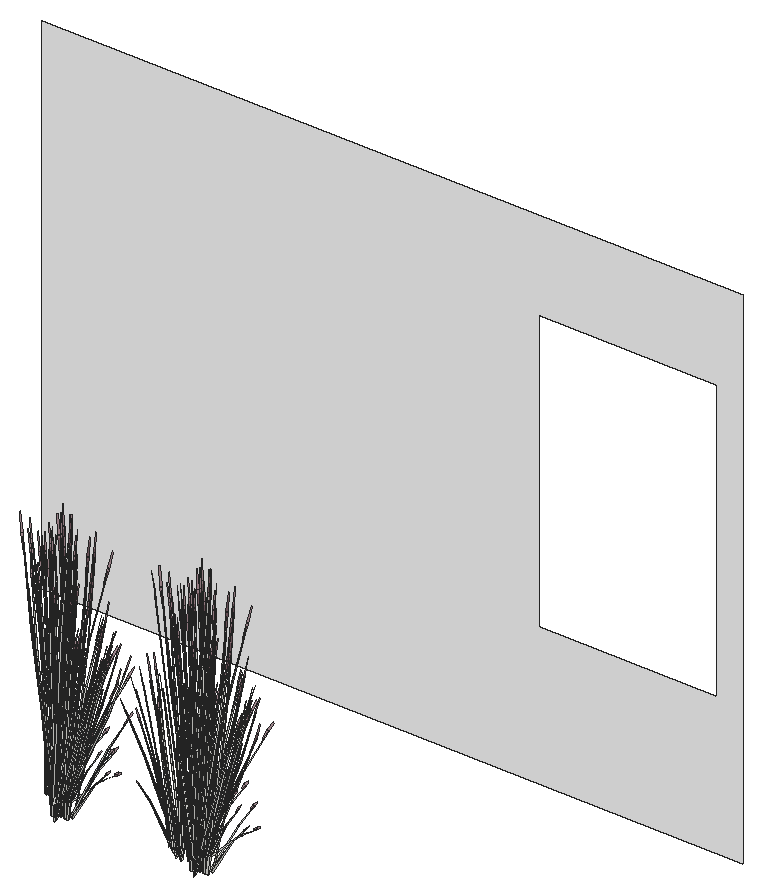
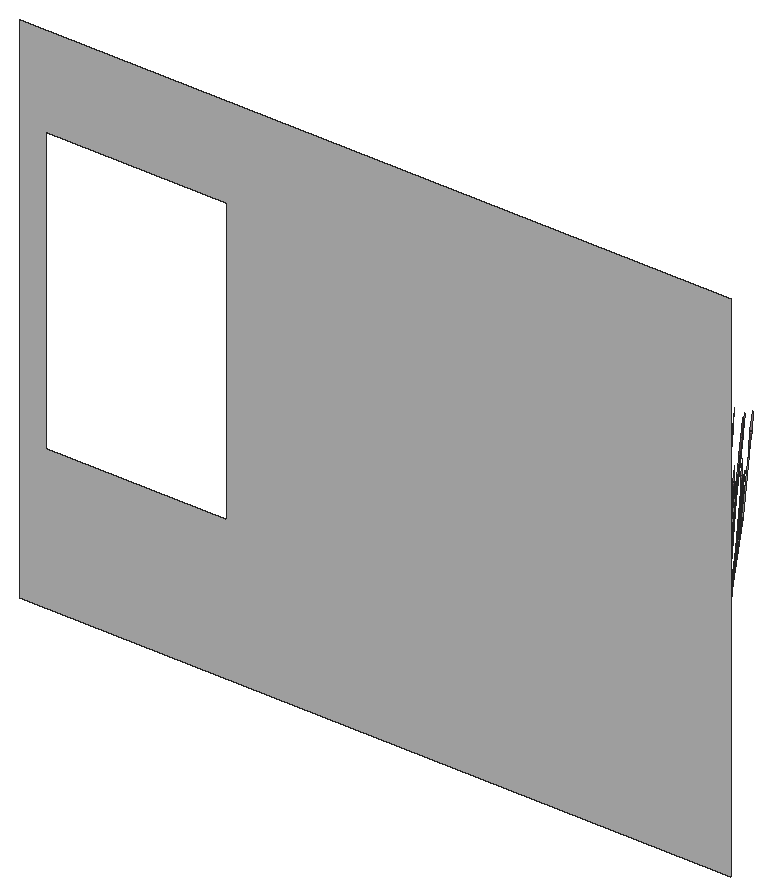
# SketchUp Ruby script. Lengths in inches.
U = 1.inch
M = Sketchup.active_model
def pt(a) = Geom::Point3d.new(a.map { |v| v * U })
def face(e, loops, mat)
  f = e.add_face(loops[0].map { |a| pt(a) })
  loops[1..].each { |l| e.add_face(l.map { |a| pt(a) }).erase! }
  f.material = f.back_material = mat if mat
  f
end
# faces: each face lists its corners as indices into pts; further lists are holes
def faces(e, pts, list, mat = nil) = list.each { |f| face(e, (f[0].is_a?(Array) ? f : [f]).map { |l| l.map { |i| pts[i] } }, mat) }
# xy, xz, yz: faces in a plane at the given z, y or x. An outline is a flat list of corners, or four numbers for a rectangle; further outlines are holes
def ring(l) = l.size == 4 ? [[l[0], l[1]], [l[2], l[1]], [l[2], l[3]], [l[0], l[3]]] : l.each_slice(2).to_a
def flat(e, list, mat, &to3) = list.each { |f| face(e, (f[0].is_a?(Array) ? f : [f]).map { |l| ring(l).map { |u, v| to3.(u, v) } }, mat) }
def xy(e, z, list, mat = nil) = flat(e, list, mat) { |x, y| [x, y, z] }
def xz(e, y, list, mat = nil) = flat(e, list, mat) { |x, z| [x, y, z] }
def yz(e, x, list, mat = nil) = flat(e, list, mat) { |y, z| [x, y, z] }
def lines(e, pts, list) = list.each { |a, b| e.add_line(pt(pts[a]), pt(pts[b])) }
# prism: a flat outline (further loops are holes) pulled along v
def prism(e, loops, v, mat = nil)
  f = face(e, loops, mat); d = Geom::Vector3d.new(v.map { |x| x * U })
  f.pushpull(f.normal.samedirection?(d) ? d.length : -d.length)
end
def box(e, o, s, mat = nil) = prism(e, [[o, [o[0] + s[0], o[1], o[2]], [o[0] + s[0], o[1] + s[1], o[2]], [o[0], o[1] + s[1], o[2]]]], [0, 0, s[2]], mat)
def at(x, y, z, deg = 0) = Geom::Transformation.translation(pt([x, y, z])) * Geom::Transformation.rotation(ORIGIN, Z_AXIS, deg.degrees)
def axes(o, x, y, z) = Geom::Transformation.new([*x, 0, *y, 0, *z, 0, *pt(o).to_a, 1])
def part(name) = M.definitions.add(name)
# library, detail: a bought-in or finely detailed component or shape, given as its bounding box
def library(name, o, s) = part(name).tap { |d| box(d.entities, o, s) }
def detail(e, o, s) = box(e.add_group.entities, o, s)
def put(e, d, t, mat = nil) = e.add_instance(d, t).tap { |i| i.material = mat if mat }
def group(e, t, mat = nil) = e.add_group.tap { |g| g.transformation = t; g.material = mat if mat }.entities
root = M.entities
M.materials.add("LightPink_Translucent").color = [144, 107, 117]
M.materials["LightPink_Translucent"].alpha = 0.75
M.materials.add("M00_Soft_Cloud").color = [255, 255, 255]
c1 = part("blade")
p = [[2.15,0.21,22],[0,0.17,0],[0.09,0.45,0],[2.18,0.31,22],[2.29,0.31,22],[0.38,0.45,0],
  [2.48,0.24,33],[2.49,0.24,33],[2.48,0.22,33]]
faces(c1.entities,p,[[0,1,2,3],[4,5,2,3],[6,3,4,7],[8,0,3,6]])
c2 = part("seeds")
p = [[0.3,-0.1,1.38],[-0.01,-0.03,1.59],[-0.01,-0.03,0.03],[0.14,-0.07,-0.07],[0.29,-0.03,3],[0.15,0.01,3.11]]
faces(c2.entities,p,[[0,1,2,3],[1,0,4,5]],"LightPink_Translucent")
c3 = part("blade with seeds")
put(c3.entities,c1,at(0,0,0))
put(c3.entities,c2,axes([2.4,0.25,30.99],[1.5799,-0.05474,1.17369],[-0.12525,1.92788,0.29478],[-0.07173,-0.02425,1.56792]))
xz(root,72.98,[[[234,0,399,120],[351,33,393,99]]],"M00_Soft_Cloud")
put(root,c3,axes([286.19,11.56,-3.97],[0.17848,0.53243,-0.30978],[-0.70886,0.15119,0.30978],[0.1429,0.0614,1.38974]))
put(root,c3,axes([318.98,11.56,-3.97],[0.17848,0.53243,-0.30978],[-0.70886,0.15119,0.30978],[0.1429,0.0614,1.38974]))
put(root,c3,axes([287.41,13.6875,-1.27],[0.27906,0.41663,0.0643],[-0.50888,0.20393,0.50621],[0.22432,-0.04024,0.77189]))
put(root,c3,axes([320.2,13.6875,-1.27],[0.27906,0.41663,0.0643],[-0.50888,0.20393,0.50621],[0.22432,-0.04024,0.77189]))
put(root,c3,axes([284.76,12.75,-3.62],[-0.96033,-0.12874,0.49198],[0.19544,-0.7271,0.19306],[0.14034,0.07021,1.70813]))
put(root,c3,axes([317.56,12.75,-3.62],[-0.96033,-0.12874,0.49198],[0.19544,-0.7271,0.19306],[0.14034,0.07021,1.70813]))
put(root,c3,axes([287.36,13.54,-1.27],[-0.21466,0.55714,0.48003],[-0.70573,-0.19051,0.3958],[0.27753,-0.03348,0.9933]))
put(root,c3,axes([320.15,13.54,-1.27],[-0.21466,0.55714,0.48003],[-0.70573,-0.19051,0.3958],[0.27753,-0.03348,0.9933]))
put(root,c3,axes([284,14.55,-3.8],[-0.24791,-0.5268,0],[0.70791,-0.18448,0],[0,0,1.54371]))
put(root,c3,axes([316.79,14.55,-3.8],[-0.24791,-0.5268,0],[0.70791,-0.18448,0],[0,0,1.54371]))
put(root,c3,axes([283.52,14.05,-3.38],[-0.14658,0.54532,0.1448],[-0.71613,-0.09466,-0.41347],[-0.13033,-0.05599,1.26744]))
put(root,c3,axes([316.32,14.05,-3.38],[-0.14658,0.54532,0.1448],[-0.71613,-0.09466,-0.41347],[-0.13033,-0.05599,1.26744]))
put(root,c3,axes([313.54,12.63,-0.95],[0.63144,0.17046,0.35414],[-0.18417,0.49731,-0.4572],[-0.25423,0.0456,0.87481]))
put(root,c3,axes([284.93,14.47,-3.82],[0.79769,-0.20732,-0.19198],[0.2803,0.59721,0.00008],[0.08805,-0.02292,1.73897]))
put(root,c3,axes([317.72,14.47,-3.82],[0.79769,-0.20732,-0.19198],[0.2803,0.59721,0.00008],[0.08805,-0.02292,1.73897]))
put(root,c3,axes([285.2,14.72,-3.53],[0.21949,-0.60727,0.17642],[0.8032,0.17185,0.35086],[-0.13875,0.00296,1.60407]))
put(root,c3,axes([318,14.72,-3.53],[0.21949,-0.60727,0.17642],[0.8032,0.17185,0.35086],[-0.13875,0.00296,1.60407]))
put(root,c3,axes([285.02,13.34,-3.79],[0.53038,0.39469,0],[-0.53038,0.39469,0],[0,0,1.69266]))
put(root,c3,axes([317.8125,13.34,-3.79],[0.53038,0.39469,0],[-0.53038,0.39469,0],[0,0,1.69266]))
put(root,c3,axes([314.8,12.6,-2.66],[0.21597,-0.08839,1.77064],[0.07448,0.61717,0.13857],[-0.4678,0.08189,0.63284]))
put(root,c3,axes([286.46,13.17,-3.53],[-0.59697,-0.44509,0.17642],[0.60159,-0.4317,0.35086],[-0.06593,0.0909,1.60407]))
put(root,c3,axes([319.25,13.17,-3.53],[-0.59697,-0.44509,0.17642],[0.60159,-0.4317,0.35086],[-0.06593,0.0909,1.60407]))
put(root,c3,axes([285.35,12.5,-3.94],[0.79037,0.10018,-0.62353],[-0.16679,0.61794,-0.16365],[0.23587,0.07488,1.37633]))
put(root,c3,axes([318.14,12.5,-3.94],[0.79037,0.10018,-0.62353],[-0.16679,0.61794,-0.16365],[0.23587,0.07488,1.37633]))
put(root,c3,axes([288.84,13.58,-3.23],[-0.46945,0.10088,1.1486],[0.22097,-0.4169,0.84392],[0.24904,0.02853,0.25299]))
put(root,c3,axes([321.64,13.58,-3.23],[-0.46945,0.10088,1.1486],[0.22097,-0.4169,0.84392],[0.24904,0.02853,0.25299]))
put(root,c3,axes([283.82,14.78,-3.8],[-0.76598,-0.27433,0],[0.36864,-0.57001,0],[0,0,1.62707]))
put(root,c3,axes([316.62,14.78,-3.8],[-0.76598,-0.27433,0],[0.36864,-0.57001,0],[0,0,1.62707]))
put(root,c3,axes([284.46,14.05,-3.54],[-0.74193,-0.49181,-0.25192],[0.6243,-0.55226,0.5513],[-0.19979,0.05753,1.68216]))
put(root,c3,axes([317.25,14.05,-3.54],[-0.74193,-0.49181,-0.25192],[0.6243,-0.55226,0.5513],[-0.19979,0.05753,1.68216]))
put(root,c3,axes([282.51,15,-3.52],[0.7111,0.30552,0.49651],[-0.42504,0.54784,0],[-0.16196,-0.06958,1.57504]))
put(root,c3,axes([315.3,15,-3.52],[0.7111,0.30552,0.49651],[-0.42504,0.54784,0],[-0.16196,-0.06958,1.57504]))
put(root,c3,axes([285.01,12.88,-3.28],[0.36864,-0.55059,0.44739],[0.76598,0.26498,-0.21531],[0,0.12692,1.43643]))
put(root,c3,axes([317.81,12.88,-3.28],[0.36864,-0.55059,0.44739],[0.76598,0.26498,-0.21531],[0,0.12692,1.43643]))
put(root,c3,axes([288.625,15.34,-1.29],[-0.0687,-0.05349,1.77383],[0.15029,-0.57341,-0.16761],[0.27062,-0.03664,0.31391]))
put(root,c3,axes([312.48,13.02,-1.28],[-0.12407,0.07933,1.74944],[0.01055,0.57963,-0.27667],[-0.2844,0.07538,0.14031]))
put(root,c3,axes([284.87,13.2,-3.71],[0,0.70667,-0.05637],[-0.95008,0,0],[0,0.02221,1.79368]))
put(root,c3,axes([317.66,13.2,-3.71],[0,0.70667,-0.05637],[-0.95008,0,0],[0,0.02221,1.79368]))
put(root,c3,axes([313.31,12.94,-1.32],[-0.20584,0.55581,-0.51099],[-0.70573,-0.19051,-0.3958],[-0.28414,0.05097,0.97773]))
put(root,c3,axes([313.27,12.46,-0.97],[0.38229,0.5533,-0.1216],[-0.6785,0.2719,-0.67495],[-0.28593,0.073,1.02557]))
put(root,c3,axes([284.94,12.7,-3.79],[0.45644,0.51287,-0.44739],[-0.69137,0.36116,0.21531],[0.14771,0.06346,1.43643]))
put(root,c3,axes([317.73,12.7,-3.79],[0.45644,0.51287,-0.44739],[-0.69137,0.36116,0.21531],[0.14771,0.06346,1.43643]))
put(root,c3,axes([288.03,14.87,-2.07],[-0.14542,-0.51365,-0.03492],[0.68734,-0.11809,-0.15832],[0.14353,0.03256,0.52218]))
put(root,c3,axes([320.82,14.87,-2.07],[-0.14542,-0.51365,-0.03492],[0.68734,-0.11809,-0.15832],[0.14353,0.03256,0.52218]))
put(root,c3,axes([314.89,15.32,-3.625],[-0.47504,0.61229,0],[-0.79476,-0.34146,-0.51607],[-0.18101,-0.07777,1.63711]))
put(root,c3,axes([286.25,14.85,-0.97],[0.04068,-0.62141,-0.1216],[0.77029,0.01698,-0.67495],[0.29667,0.04317,1.02557]))
put(root,c3,axes([319.04,14.85,-0.97],[0.04068,-0.62141,-0.1216],[0.77029,0.01698,-0.67495],[0.29667,0.04317,1.02557]))
put(root,c3,axes([286.95,13.19,-3.52],[0,-0.61104,0.49651],[0.85008,0,0],[0,0.13917,1.57504]))
put(root,c3,axes([319.74,13.19,-3.52],[0,-0.61104,0.49651],[0.85008,0,0],[0,0.13917,1.57504]))
put(root,c3,axes([284.82,13.65,-3.28],[0.82508,-0.03772,0.44739],[0.07462,0.62614,-0.21531],[-0.14771,0.06346,1.43643]))
put(root,c3,axes([317.61,13.65,-3.28],[0.82508,-0.03772,0.44739],[0.07462,0.62614,-0.21531],[-0.14771,0.06346,1.43643]))
put(root,c3,axes([285.33,13.01,-3.38],[0.70791,-0.1782,0.1448],[0.24791,0.50885,-0.41347],[0,0.11199,1.26744]))
put(root,c3,axes([318.125,13.01,-3.38],[0.70791,-0.1782,0.1448],[0.24791,0.50885,-0.41347],[0,0.11199,1.26744]))
put(root,c3,axes([286.13,14.61,-0.95],[-0.43232,-0.38257,0.35414],[0.49364,-0.36215,-0.4572],[0.25081,0.0551,0.87481]))
put(root,c3,axes([318.92,14.61,-0.95],[-0.43232,-0.38257,0.35414],[0.49364,-0.36215,-0.4572],[0.25081,0.0551,0.87481]))
put(root,c3,axes([284.08,13.95,-3.79],[-0.82508,0.03772,-0.44739],[-0.07462,-0.62614,0.21531],[-0.14771,0.06346,1.43643]))
put(root,c3,axes([316.875,13.95,-3.79],[-0.82508,0.03772,-0.44739],[-0.07462,-0.62614,0.21531],[-0.14771,0.06346,1.43643]))
put(root,c3,axes([287.96,14.25,-3.41],[-0.18299,-0.15028,1.43002],[0.23809,-0.49714,-0.30754],[0.37023,0.06735,0.61141]))
put(root,c3,axes([284.69,14.8,-3.8],[0.76598,0.27433,0],[-0.36864,0.57001,0],[0,0,1.74954]))
put(root,c3,axes([317.49,14.8,-3.8],[0.76598,0.27433,0],[-0.36864,0.57001,0],[0,0,1.74954]))
put(root,c3,axes([286.92,14.48,-1.28],[0.16299,-0.01033,1.74944],[0.44707,-0.47471,-0.27667],[0.28992,0.06266,0.14031]))
put(root,c3,axes([319.71,14.48,-1.28],[0.16299,-0.01033,1.74944],[0.44707,-0.47471,-0.27667],[0.28992,0.06266,0.14031]))
put(root,c3,axes([285,15.4,-3.81],[-0.46912,-0.61443,-0.05142],[0.79476,-0.34146,0.51607],[-0.19584,0.0585,1.6363]))
put(root,c3,axes([317.79,15.4,-3.81],[-0.46912,-0.61443,-0.05142],[0.79476,-0.34146,0.51607],[-0.19584,0.0585,1.6363]))
put(root,c3,axes([284.83,13.92,-3.38],[0.56134,0.36712,0.1448],[-0.46823,0.41419,-0.41347],[-0.13033,0.05599,1.26744]))
put(root,c3,axes([317.625,13.92,-3.38],[0.56134,0.36712,0.1448],[-0.46823,0.41419,-0.41347],[-0.13033,0.05599,1.26744]))
put(root,c3,axes([313.19,14.01,-1.27],[-0.18844,-0.56237,0.48003],[0.73919,-0.0976,0.3958],[-0.21785,0.13226,0.9933]))
put(root,c3,axes([313.05,13.9,-1.27],[-0.52161,-0.25698,0.0643],[0.30368,-0.36595,0.50621],[-0.16723,0.11831,0.77189]))
put(root,c3,axes([313.28,13.23,-2.125],[0.26363,-0.12925,1.71376],[0.22195,0.59723,0.13857],[-0.41388,0.13498,0.73262]))
put(root,c3,axes([286.28,14.55,-1.02],[0.75952,0.01471,-0.71045],[-0.05101,0.61953,0.08574],[0.32177,0.06538,1.00501]))
put(root,c3,axes([285.43,15.05,-3.52],[0.7111,-0.30552,0.49651],[0.42504,0.54784,0],[-0.16196,0.06958,1.57504]))
put(root,c3,axes([318.22,15.05,-3.52],[0.7111,-0.30552,0.49651],[0.42504,0.54784,0],[-0.16196,0.06958,1.57504]))
put(root,c3,axes([284.42,14.57,-3.71],[0.33034,0.70197,-0.06012],[-0.94388,0.24598,0],[0.01154,0.02451,1.72173]))
put(root,c3,axes([317.21,14.57,-3.71],[0.33034,0.70197,-0.06012],[-0.94388,0.24598,0],[0.01154,0.02451,1.72173]))
put(root,c3,axes([284.78,15.32,-3.97],[-0.70886,-0.15119,-0.30978],[0.17848,-0.53243,0.30978],[-0.1429,0.0614,1.38974]))
put(root,c3,axes([317.58,15.32,-3.97],[-0.70886,-0.15119,-0.30978],[0.17848,-0.53243,0.30978],[-0.1429,0.0614,1.38974]))
put(root,c3,axes([312.46,14.24,-3.41],[0.26405,0.05016,1.43002],[0.17019,0.51235,-0.30754],[-0.35868,0.0959,0.61141]))
put(root,c3,axes([313.65,13.83,-0.95],[0.66138,-0.08733,0.35414],[0.17464,0.49921,-0.4572],[-0.18953,0.13408,0.87481]))
put(root,c3,axes([287.52,13.29,-3.625],[0.95008,0,0],[0,0.68292,-0.51607],[0,0.15554,1.63711]))
put(root,c3,axes([320.32,13.29,-3.625],[0.95008,0,0],[0,0.68292,-0.51607],[0,0.15554,1.63711]))
put(root,c3,axes([311.1,13.6,-1.29],[0.09697,0.01639,1.77383],[0.29997,0.53988,-0.16761],[-0.1985,0.1417,0.31391]))
put(root,c3,axes([287.14,13.64,-3.8],[-0.94962,-0.00489,-0.04976],[0,-0.68292,0.49943],[-0.02984,0.15546,1.58352]))
put(root,c3,axes([319.9375,13.64,-3.8],[-0.94962,-0.00489,-0.04976],[0,-0.68292,0.49943],[-0.02984,0.15546,1.58352]))
put(root,c3,axes([285.09,13.05,-3.33],[0.85568,0.29155,-0.29095],[-0.41201,0.61537,-0.50002],[0.02689,0.15109,1.59708]))
put(root,c3,axes([317.88,13.05,-3.33],[0.85568,0.29155,-0.29095],[-0.41201,0.61537,-0.50002],[0.02689,0.15109,1.59708]))
put(root,c3,axes([311.91,15.32,-3.23],[0.31665,-0.27694,1.1486],[0.12495,0.43841,0.84392],[-0.22883,0.0785,0.25299]))
put(root,c3,axes([286.74,14.81,-1.47],[0.43232,0.38257,-0.35414],[-0.49364,0.36215,0.4572],[0.25081,0.0551,0.87481]))
put(root,c3,axes([319.53,14.81,-1.47],[0.43232,0.38257,-0.35414],[-0.49364,0.36215,0.4572],[0.25081,0.0551,0.87481]))
put(root,c3,axes([286.95,13.74,-3.97],[-0.53038,0.38124,-0.30978],[-0.53038,-0.38124,0.30978],[0,0.1228,1.38974]))
put(root,c3,axes([319.74,13.74,-3.97],[-0.53038,0.38124,-0.30978],[-0.53038,-0.38124,0.30978],[0,0.1228,1.38974]))
put(root,c3,axes([284.66,13.78,-3.33],[0.08854,0.69723,-0.29095],[-0.92215,0.04216,-0.50002],[-0.16238,0.09287,1.59708]))
put(root,c3,axes([317.46,13.78,-3.33],[0.08854,0.69723,-0.29095],[-0.92215,0.04216,-0.50002],[-0.16238,0.09287,1.59708]))
put(root,c3,axes([286.52,14.95,-1.27],[-0.03826,0.46465,0.0643],[-0.57772,-0.01274,0.50621],[0.2213,0.04862,0.77189]))
put(root,c3,axes([319.3125,14.95,-1.27],[-0.03826,0.46465,0.0643],[-0.57772,-0.01274,0.50621],[0.2213,0.04862,0.77189]))
put(root,c3,axes([285,13.51,-3.79],[-0.36864,0.55059,-0.44739],[-0.76598,-0.26498,0.21531],[0,0.12692,1.43643]))
put(root,c3,axes([317.79,13.51,-3.79],[-0.36864,0.55059,-0.44739],[-0.76598,-0.26498,0.21531],[0,0.12692,1.43643]))
put(root,c3,axes([313.11,14.12,-1.47],[-0.66138,0.08733,-0.35414],[-0.17464,-0.49921,0.4572],[-0.18953,0.13408,0.87481]))
put(root,c3,axes([286.57,14.81,-1.27],[-0.56024,0.40262,0.48003],[-0.48318,-0.42758,0.3958],[0.26285,0.07427,0.9933]))
put(root,c3,axes([319.37,14.81,-1.27],[-0.56024,0.40262,0.48003],[-0.48318,-0.42758,0.3958],[0.26285,0.07427,0.9933]))
put(root,c3,axes([312.14,15.24,-0.35],[0.67048,0.16311,-0.06488],[-0.20625,0.50201,-0.29416],[-0.10966,0.07622,0.97024]))
put(root,c3,axes([284.11,14.3125,-3.94],[-0.51177,0.45928,-0.62353],[-0.63575,-0.41646,-0.16365],[-0.20507,0.11457,1.37633]))
put(root,c3,axes([316.9,14.3125,-3.94],[-0.51177,0.45928,-0.62353],[-0.63575,-0.41646,-0.16365],[-0.20507,0.11457,1.37633]))
put(root,c3,axes([284.79,15.27,-0.95],[-0.11735,-0.49217,0.35414],[0.67083,-0.12996,-0.4572],[0.18018,0.14104,0.87481]))
put(root,c3,axes([317.58,15.27,-0.95],[-0.11735,-0.49217,0.35414],[0.67083,-0.12996,-0.4572],[0.18018,0.14104,0.87481]))
put(root,c3,axes([285.02,15.09,-3.67],[0.95122,0.19861,0.30756],[-0.23797,0.7099,-0.36492],[-0.15744,0.08885,1.64885]))
put(root,c3,axes([317.8125,15.09,-3.67],[0.95122,0.19861,0.30756],[-0.23797,0.7099,-0.36492],[-0.15744,0.08885,1.64885]))
put(root,c3,axes([284.95,15.57,-3.98],[-0.7111,0.30552,-0.49651],[-0.42504,-0.54784,0],[-0.16196,0.06958,1.57504]))
put(root,c3,axes([317.74,15.57,-3.98],[-0.7111,0.30552,-0.49651],[-0.42504,-0.54784,0],[-0.16196,0.06958,1.57504]))
put(root,c3,axes([287.3125,13.76,-3.98],[0,0.61104,-0.49651],[-0.85008,0,0],[0,0.13917,1.57504]))
put(root,c3,axes([320.11,13.76,-3.98],[0,0.61104,-0.49651],[-0.85008,0,0],[0,0.13917,1.57504]))
put(root,c3,axes([285.1875,13.83,-2.125],[-0.28223,-0.10528,1.71376],[0.58406,-0.44165,0.13857],[0.36402,0.19924,0.73262]))
put(root,c3,axes([317.98,13.83,-2.125],[-0.28223,-0.10528,1.71376],[0.58406,-0.44165,0.13857],[0.36402,0.19924,0.73262]))
put(root,c3,axes([285.24,12.44,-1.53],[-0.65655,-0.31748,1.38283],[0.69326,-0.49431,0.59665],[0.21183,0.29789,1.33663]))
put(root,c3,axes([318.04,12.44,-1.53],[-0.65655,-0.31748,1.38283],[0.69326,-0.49431,0.59665],[0.21183,0.29789,1.33663]))
put(root,c3,axes([313.3,13.78,-0.97],[0.70283,0.33692,-0.1216],[-0.40491,0.48793,-0.67495],[-0.19857,0.16961,1.02557]))
put(root,c3,axes([286.23,15.02,-3.23],[-0.4278,-0.1757,1.1486],[0.5524,-0.17852,0.84392],[0.14899,0.15122,0.25299]))
put(root,c3,axes([319.03,15.02,-3.23],[-0.4278,-0.1757,1.1486],[0.5524,-0.17852,0.84392],[0.14899,0.15122,0.25299]))
put(root,c3,axes([284.73,15.53,-0.97],[0.45276,-0.52302,-0.1216],[0.65568,0.30132,-0.67495],[0.22792,0.14777,1.02557]))
put(root,c3,axes([317.52,15.53,-0.97],[0.45276,-0.52302,-0.1216],[0.65568,0.30132,-0.67495],[0.22792,0.14777,1.02557]))
put(root,c3,axes([314.25,13.63,-2.125],[0.18977,-0.18775,1.71376],[0.47917,0.50677,0.13857],[-0.32866,0.23079,0.73262]))
put(root,c3,axes([313.65,14.18,-1.32],[0.19519,0.55794,-0.51099],[-0.73919,0.0976,-0.3958],[-0.21183,0.14986,0.97773]))
put(root,c3,axes([281.74,14.82,-0.95],[0.5141,-0.32171,0.35414],[0.48666,0.36734,-0.4572],[-0.07405,0.18664,0.87481]))
put(root,c3,axes([314.54,14.82,-0.95],[0.5141,-0.32171,0.35414],[0.48666,0.36734,-0.4572],[-0.07405,0.18664,0.87481]))
put(root,c3,axes([285.6,15.47,-3.625],[0.47504,0.61229,0],[-0.79476,0.34146,-0.51607],[-0.18101,0.07777,1.63711]))
put(root,c3,axes([318.39,15.47,-3.625],[0.47504,0.61229,0],[-0.79476,0.34146,-0.51607],[-0.18101,0.07777,1.63711]))
put(root,c3,axes([284.14,15.96,-1.29],[0.00225,-0.07398,1.77383],[0.65113,-0.32638,-0.16761],[0.22617,0.1165,0.31391]))
put(root,c3,axes([316.93,15.96,-1.29],[0.00225,-0.07398,1.77383],[0.65113,-0.32638,-0.16761],[0.22617,0.1165,0.31391]))
put(root,c3,axes([286.35,15.68,-4.51],[0.05536,-0.08822,1.76342],[0.69692,-0.25981,-0.26939],[0.21129,0.13447,0.30037]))
put(root,c3,axes([319.15,15.68,-4.51],[0.05536,-0.08822,1.76342],[0.69692,-0.25981,-0.26939],[0.21129,0.13447,0.30037]))
put(root,c3,axes([285.19,13.05,-3.16],[-0.02076,-0.57531,1.41272],[0.93937,0.14913,0.59816],[-0.22217,0.31481,1.3335]))
put(root,c3,axes([317.98,13.05,-3.16],[-0.02076,-0.57531,1.41272],[0.93937,0.14913,0.59816],[-0.22217,0.31481,1.3335]))
put(root,c3,axes([285.43,13.67,-3.91],[0.2786,0.55945,-0.69212],[-0.80253,0.20149,-0.18165],[0.03079,0.18945,1.52773]))
put(root,c3,axes([318.23,13.67,-3.91],[0.2786,0.55945,-0.69212],[-0.80253,0.20149,-0.18165],[0.03079,0.18945,1.52773]))
put(root,c3,axes([281.28,15.11,-1.27],[-0.62439,-0.02847,0.0643],[0.01712,-0.42991,0.50621],[-0.06534,0.16468,0.77189]))
put(root,c3,axes([314.07,15.11,-1.27],[-0.62439,-0.02847,0.0643],[0.01712,-0.42991,0.50621],[-0.06534,0.16468,0.77189]))
put(root,c3,axes([312.75,15.6,-4.51],[0.10192,0.06105,1.76342],[0.17281,0.56562,-0.26939],[-0.22588,0.12062,0.30037]))
put(root,c3,axes([281.48,15.15,-1.27],[-0.54105,-0.41691,0.48003],[0.57458,-0.35956,0.3958],[-0.0998,0.1956,0.9933]))
put(root,c3,axes([314.27,15.15,-1.27],[-0.54105,-0.41691,0.48003],[0.57458,-0.35956,0.3958],[-0.0998,0.1956,0.9933]))
put(root,c3,axes([285.27,15.27,-1.32],[0.74975,-0.14525,-0.51099],[0.13115,0.55007,-0.3958],[0.20138,0.15763,0.97773]))
put(root,c3,axes([318.06,15.27,-1.32],[0.74975,-0.14525,-0.51099],[0.13115,0.55007,-0.3958],[0.20138,0.15763,0.97773]))
put(root,c3,axes([283.1875,15.35,-0.95],[0.22906,-0.4699,0.35414],[0.66828,0.13705,-0.4572],[0.06128,0.18919,0.87481]))
put(root,c3,axes([315.98,15.35,-0.95],[0.22906,-0.4699,0.35414],[0.66828,0.13705,-0.4572],[0.06128,0.18919,0.87481]))
put(root,c3,axes([286.3,15.82,-3.33],[-0.48723,-0.01916,1.0506],[0.32177,-0.40701,0.58006],[0.19248,0.1446,0.8241]))
put(root,c3,axes([319.09,15.82,-3.33],[-0.48723,-0.01916,1.0506],[0.32177,-0.40701,0.58006],[0.19248,0.1446,0.8241]))
put(root,c3,axes([284.9,15.72,-1.27],[-0.34533,0.38816,0.0643],[-0.49176,-0.22599,0.50621],[0.15898,0.12445,0.77189]))
put(root,c3,axes([317.69,15.72,-1.27],[-0.34533,0.38816,0.0643],[-0.49176,-0.22599,0.50621],[0.15898,0.12445,0.77189]))
put(root,c3,axes([284.09,17.03,-0.35],[0.52505,-0.35054,-0.06488],[0.48109,0.38392,-0.29416],[0.03387,0.10878,0.97024]))
put(root,c3,axes([316.88,17.03,-0.35],[0.52505,-0.35054,-0.06488],[0.48109,0.38392,-0.29416],[0.03387,0.10878,0.97024]))
put(root,c3,axes([285.04,15.61,-1.27],[-0.75571,0.14023,0.48003],[-0.13115,-0.55007,0.3958],[0.17773,0.16212,0.9933]))
put(root,c3,axes([317.84,15.61,-1.27],[-0.75571,0.14023,0.48003],[-0.13115,-0.55007,0.3958],[0.17773,0.16212,0.9933]))
put(root,c3,axes([314.11,14.09,-2.125],[0.14147,-0.21002,1.71376],[0.59349,0.43464,0.13857],[-0.26773,0.27089,0.73262]))
put(root,c3,axes([284.71,14.84,-3.41],[0.01341,-0.20255,1.43002],[0.64074,-0.22625,-0.30754],[0.1978,0.24243,0.61141]))
put(root,c3,axes([317.5,14.84,-3.41],[0.01341,-0.20255,1.43002],[0.64074,-0.22625,-0.30754],[0.1978,0.24243,0.61141]))
put(root,c3,axes([282.98,15.77,-1.27],[-0.55987,0.20767,0.0643],[-0.27403,-0.37869,0.50621],[0.05407,0.16693,0.77189]))
put(root,c3,axes([315.77,15.77,-1.27],[-0.55987,0.20767,0.0643],[-0.27403,-0.37869,0.50621],[0.05407,0.16693,0.77189]))
put(root,c3,axes([281.48,15.28,-1.47],[-0.5141,0.32171,-0.35414],[-0.48666,-0.36734,0.4572],[-0.07405,0.18664,0.87481]))
put(root,c3,axes([314.27,15.28,-1.47],[-0.5141,0.32171,-0.35414],[-0.48666,-0.36734,0.4572],[-0.07405,0.18664,0.87481]))
put(root,c3,axes([312.5,15.18,-1.28],[-0.01889,0.12092,1.74944],[0.53598,0.42065,-0.27667],[-0.14032,0.19892,0.14031]))
put(root,c3,axes([281.42,14.91,-0.6],[0.83505,0.03027,-0.13498],[-0.02282,0.57322,-0.74919],[-0.05801,0.22077,1.13838]))
put(root,c3,axes([314.21,14.91,-0.6],[0.83505,0.03027,-0.13498],[-0.02282,0.57322,-0.74919],[-0.05801,0.22077,1.13838]))
put(root,c3,axes([282.96,15.55,-0.97],[0.74352,-0.28449,-0.1216],[0.36538,0.50492,-0.67495],[0.0981,0.21277,1.02557]))
put(root,c3,axes([315.76,15.55,-0.97],[0.74352,-0.28449,-0.1216],[0.36538,0.50492,-0.67495],[0.0981,0.21277,1.02557]))
put(root,c3,axes([283.18,15.73,-0.9375],[-0.74868,-0.15974,0.53283],[0.25601,-0.52518,0.43934],[0.04499,0.20653,1.10256]))
put(root,c3,axes([315.97,15.73,-0.9375],[-0.74868,-0.15974,0.53283],[0.25601,-0.52518,0.43934],[0.04499,0.20653,1.10256]))
put(root,c3,axes([281.8,16.53,-3.23],[-0.01966,-0.36332,1.1486],[0.49135,0.25914,0.84392],[-0.09663,0.17317,0.25299]))
put(root,c3,axes([314.6,16.53,-3.23],[-0.01966,-0.36332,1.1486],[0.49135,0.25914,0.84392],[-0.09663,0.17317,0.25299]))
put(root,c3,axes([283.1,15.66,-4.51],[0.12297,-0.03325,1.76342],[0.73967,0.18301,-0.26939],[0.02163,0.20626,0.30037]))
put(root,c3,axes([315.89,15.66,-4.51],[0.12297,-0.03325,1.76342],[0.73967,0.18301,-0.26939],[0.02163,0.20626,0.30037]))
put(root,c3,axes([281.99,15.125,-1],[0.54391,0.41056,-0.5672],[-0.57458,0.35956,-0.43934],[-0.08276,0.2086,1.08528]))
put(root,c3,axes([314.78,15.125,-1],[0.54391,0.41056,-0.5672],[-0.57458,0.35956,-0.43934],[-0.08276,0.2086,1.08528]))
put(root,c3,axes([281.4,15.74,-3.18],[0.69024,-0.1082,0.06507],[0.15868,0.43593,-0.86304],[-0.04376,0.22067,0.7736]))
put(root,c3,axes([314.19,15.74,-3.18],[0.69024,-0.1082,0.06507],[0.15868,0.43593,-0.86304],[-0.04376,0.22067,0.7736]))
put(root,c3,axes([283.6,15.52,-1.32],[0.7469,0.15318,-0.51099],[-0.25601,0.52518,-0.3958],[0.06849,0.21144,0.97773]))
put(root,c3,axes([316.39,15.52,-1.32],[0.7469,0.15318,-0.51099],[-0.25601,0.52518,-0.3958],[0.06849,0.21144,0.97773]))
put(root,c3,axes([284.02,14.4375,-2.125],[-0.17368,-0.19618,1.71376],[0.80256,-0.16516,0.13857],[0.18139,0.30799,0.73262]))
put(root,c3,axes([316.82,14.4375,-2.125],[-0.17368,-0.19618,1.71376],[0.80256,-0.16516,0.13857],[0.18139,0.30799,0.73262]))
put(root,c3,axes([283.26,15.84,-1.47],[-0.22906,0.4699,-0.35414],[-0.66828,-0.13705,0.4572],[0.06128,0.18919,0.87481]))
put(root,c3,axes([316.05,15.84,-1.47],[-0.22906,0.4699,-0.35414],[-0.66828,-0.13705,0.4572],[0.06128,0.18919,0.87481]))
put(root,c3,axes([281.82,14.9375,-0.66],[-0.01977,0.56521,-0.7886],[-0.83252,-0.03796,0.09517],[-0.08786,0.23945,1.11556]))
put(root,c3,axes([314.61,14.9375,-0.66],[-0.01977,0.56521,-0.7886],[-0.83252,-0.03796,0.09517],[-0.08786,0.23945,1.11556]))
put(root,c3,axes([279.64,16.42,-1.29],[0.0862,-0.03689,1.77383],[0.71245,0.24539,-0.16761],[-0.01674,0.20431,0.31391]))
put(root,c3,axes([312.4375,16.42,-1.29],[0.0862,-0.03689,1.77383],[0.71245,0.24539,-0.16761],[-0.01674,0.20431,0.31391]))
put(root,c3,axes([282.61,14.54,-2.125],[-0.0186,-0.23452,1.71376],[0.80601,0.15558,0.13857],[-0.04985,0.33422,0.73262]))
put(root,c3,axes([315.4,14.54,-2.125],[-0.0186,-0.23452,1.71376],[0.80601,0.15558,0.13857],[-0.04985,0.33422,0.73262]))
put(root,c3,axes([283.33,15.42,-1.02],[0.36264,0.49684,-0.71045],[-0.74649,0.27689,0.08574],[0.0848,0.24006,1.00501]))
put(root,c3,axes([316.12,15.42,-1.02],[0.36264,0.49684,-0.71045],[-0.74649,0.27689,0.08574],[0.0848,0.24006,1.00501]))
put(root,c3,axes([314.02,16.2,-3.41],[0.23977,-0.09639,1.43002],[0.59198,0.29065,-0.30754],[-0.1762,0.25149,0.61141]))
put(root,c3,axes([282.79,16.68,-1.28],[0.09631,0.0984,1.74944],[0.77725,0.03866,-0.27667],[0.07816,0.217,0.14031]))
put(root,c3,axes([315.58,16.68,-1.28],[0.09631,0.0984,1.74944],[0.77725,0.03866,-0.27667],[0.07816,0.217,0.14031]))
put(root,c3,axes([281.54,15.73,-2.64],[0.01669,-0.31544,1.54345],[0.75083,0.16661,0.21329],[-0.06506,0.33618,0.72882]))
put(root,c3,axes([314.33,15.73,-2.64],[0.01669,-0.31544,1.54345],[0.75083,0.16661,0.21329],[-0.06506,0.33618,0.72882]))
